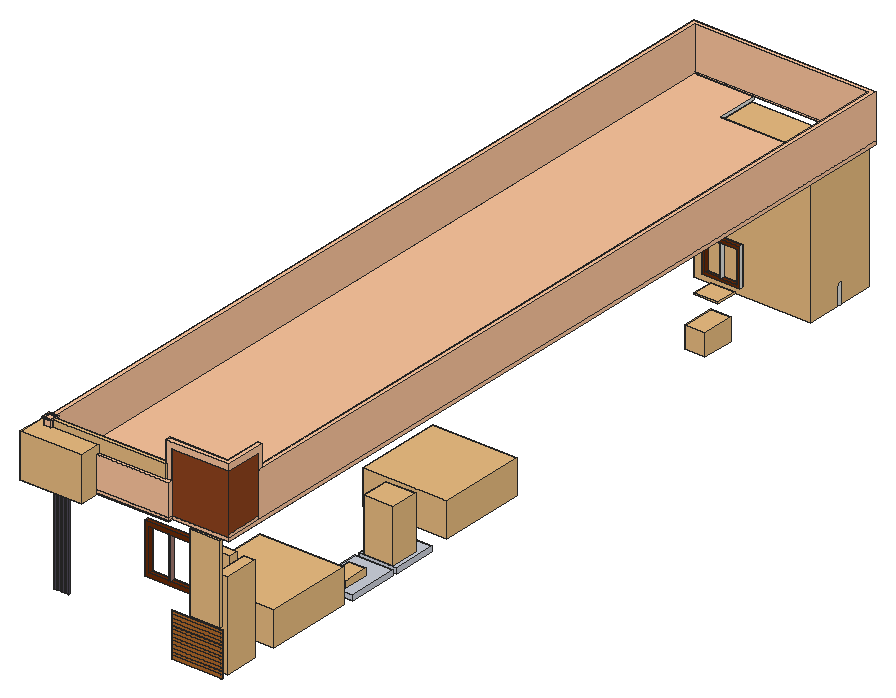
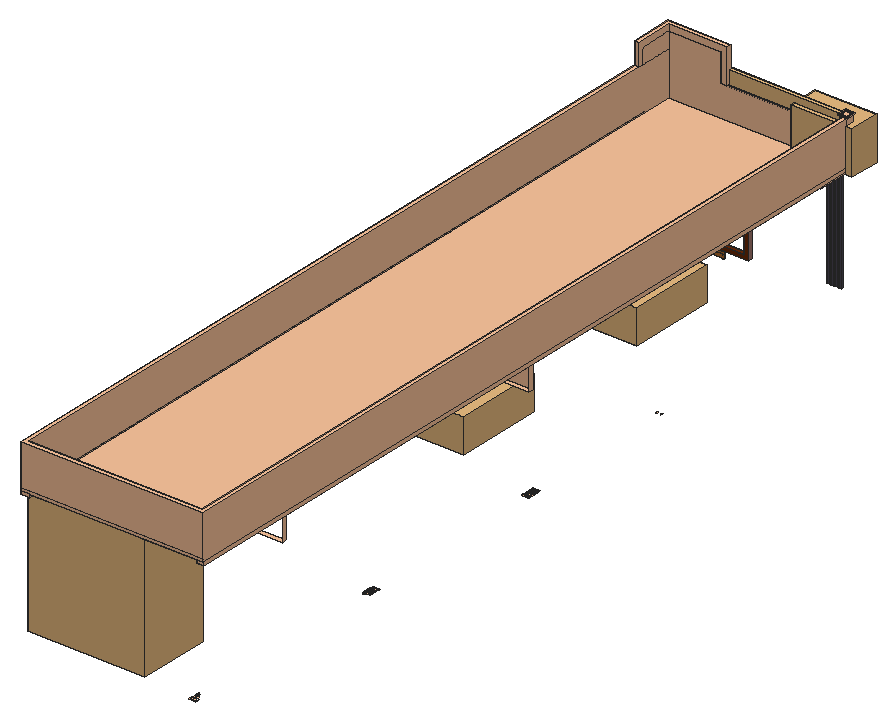
# SketchUp Ruby script. Lengths in inches.
U = 1.inch
M = Sketchup.active_model
def pt(a) = Geom::Point3d.new(a.map { |v| v * U })
def face(e, loops, mat)
  f = e.add_face(loops[0].map { |a| pt(a) })
  loops[1..].each { |l| e.add_face(l.map { |a| pt(a) }).erase! }
  f.material = f.back_material = mat if mat
  f
end
# faces: each face lists its corners as indices into pts; further lists are holes
def faces(e, pts, list, mat = nil) = list.each { |f| face(e, (f[0].is_a?(Array) ? f : [f]).map { |l| l.map { |i| pts[i] } }, mat) }
# xy, xz, yz: faces in a plane at the given z, y or x. An outline is a flat list of corners, or four numbers for a rectangle; further outlines are holes
def ring(l) = l.size == 4 ? [[l[0], l[1]], [l[2], l[1]], [l[2], l[3]], [l[0], l[3]]] : l.each_slice(2).to_a
def flat(e, list, mat, &to3) = list.each { |f| face(e, (f[0].is_a?(Array) ? f : [f]).map { |l| ring(l).map { |u, v| to3.(u, v) } }, mat) }
def xy(e, z, list, mat = nil) = flat(e, list, mat) { |x, y| [x, y, z] }
def xz(e, y, list, mat = nil) = flat(e, list, mat) { |x, z| [x, y, z] }
def yz(e, x, list, mat = nil) = flat(e, list, mat) { |y, z| [x, y, z] }
def lines(e, pts, list) = list.each { |a, b| e.add_line(pt(pts[a]), pt(pts[b])) }
# prism: a flat outline (further loops are holes) pulled along v
def prism(e, loops, v, mat = nil)
  f = face(e, loops, mat); d = Geom::Vector3d.new(v.map { |x| x * U })
  f.pushpull(f.normal.samedirection?(d) ? d.length : -d.length)
end
def box(e, o, s, mat = nil) = prism(e, [[o, [o[0] + s[0], o[1], o[2]], [o[0] + s[0], o[1] + s[1], o[2]], [o[0], o[1] + s[1], o[2]]]], [0, 0, s[2]], mat)
def at(x, y, z, deg = 0) = Geom::Transformation.translation(pt([x, y, z])) * Geom::Transformation.rotation(ORIGIN, Z_AXIS, deg.degrees)
def axes(o, x, y, z) = Geom::Transformation.new([*x, 0, *y, 0, *z, 0, *pt(o).to_a, 1])
def part(name) = M.definitions.add(name)
# library, detail: a bought-in or finely detailed component or shape, given as its bounding box
def library(name, o, s) = part(name).tap { |d| box(d.entities, o, s) }
def detail(e, o, s) = box(e.add_group.entities, o, s)
def put(e, d, t, mat = nil) = e.add_instance(d, t).tap { |i| i.material = mat if mat }
def group(e, t, mat = nil) = e.add_group.tap { |g| g.transformation = t; g.material = mat if mat }.entities
root = M.entities
M.materials.add("[0023_FireBrick]").color = [178, 34, 34]
M.materials.add("[Color A01]1").color = [163, 122, 112]
M.materials.add("[Color A02]1").color = [252, 197, 157]
M.materials.add("[Color M06]").color = [77, 72, 86]
M.materials.add("[Marble Carrara Floor Tile]").color = [204, 208, 219]
M.materials.add("[Wood Bamboo]").color = [177, 105, 43]
M.materials.add("[Wood Fence]1").color = [142, 67, 30]
M.materials.add("[Wood Veneer 02]").color = [107, 42, 7]
c1 = part("Group\#210")
box(c1.entities,[0,0,-0.3125],[36.0625,48,5.3125])
c2 = library("Group\#15",[-0.01,-1.53,0.79],[112.05,69.48,120])
c3 = library("Double bed",[0,0,0],[90.55,83.75,32.69])
c4 = part("Component\#5")
box(c4.entities,[0,-0.625,0],[48.6875,0.625,3.09])
c5 = library("P2 Single Open Right",[0,0,0],[8.91,82.42,82.52])
c6 = library("Group\#135",[0,0,0],[10.8125,33,84])
c7 = library("Squat+Toilet",[-7.87,-3.06,-5.41],[15.8,23.9,6.66])
c8 = library("My Toilet",[37.42,56.99,0],[19.17,25.6,30.6])
c9 = part("Frame upright")
box(c9.entities,[0,0,-39.22],[3.05,1.4,102],"[Color M06]")
c10 = library("Sink with faucet",[0,-0.57,-6.81],[19.24,30.87,20.8])
c11 = library("2-TABLE DE CUISSON CLC2",[-11.42,-10.04,0],[22.84,20.08,1.26])
c12 = part("Group87\#1")
xy(c12.entities,0,[[[-24,-24,24,24],[0.59,-20.0625,20.0625,20.0625],[-20.0625,-20.0625,-0.59,20.0625]]],"[Wood Veneer 02]")
xy(c12.entities,5.875,[[[-24,-24,24,24],[0.59,-20.0625,20.0625,20.0625],[-20.0625,-20.0625,-0.59,20.0625]]],"[Wood Veneer 02]")
xz(c12.entities,-24,[[-24,0,24,5.875]])
xz(c12.entities,-20.0625,[[-20.0625,0,-0.59,5.875],[0.59,0,20.0625,5.875]],"[Wood Veneer 02]")
xz(c12.entities,20.0625,[[-20.0625,0,-0.59,5.875],[0.59,0,20.0625,5.875]])
xz(c12.entities,24,[[-24,0,24,5.875]],"[Wood Veneer 02]")
yz(c12.entities,-24,[[-24,0,24,5.875]])
yz(c12.entities,-20.0625,[[-20.0625,0,20.0625,5.875]],"[Wood Veneer 02]")
yz(c12.entities,-0.59,[[-20.0625,0,20.0625,5.875]],"[Wood Veneer 02]")
yz(c12.entities,0.59,[[-20.0625,0,20.0625,5.875]])
yz(c12.entities,20.0625,[[-20.0625,0,20.0625,5.875]],"[Wood Veneer 02]")
yz(c12.entities,24,[[-24,0,24,5.875]])
c13 = library("jali",[235.9375,0,0],[159,318,2])
c14 = library("ARTIFICIAL VINES & FLOWERS",[-442.26,-138.3125,250.52],[58.45,28.9,41.46])
c15 = part("Square post")
box(c15.entities,[0,0,0],[7.1875,7.1875,27.41])
c16 = part("Component\#11")
xy(c16.entities,0,[[0,0,7.1875,7.1875]])
xy(c16.entities,12.79,[[[-0.9,-0.9,8.09,8.09],[0,0,7.1875,7.1875]],[0,0,7.1875,7.1875]])
xy(c16.entities,13.54,[[[-0.9,-0.9,8.09,8.09],[0,0,7.1875,7.1875]]])
xz(c16.entities,-0.9,[[-0.9,12.79,8.09,13.54]])
xz(c16.entities,0,[[0,0,7.1875,12.79],[0,12.79,7.1875,13.54]])
xz(c16.entities,7.1875,[[0,0,7.1875,12.79],[0,12.79,7.1875,13.54]])
xz(c16.entities,8.09,[[-0.9,12.79,8.09,13.54]])
yz(c16.entities,-0.9,[[-0.9,12.79,8.09,13.54]])
yz(c16.entities,0,[[0,0,7.1875,12.79],[0,12.79,7.1875,13.54]])
yz(c16.entities,7.1875,[[0,0,7.1875,12.79],[0,12.79,7.1875,13.54]])
yz(c16.entities,8.09,[[-0.9,12.79,8.09,13.54]])
c17 = library("Group\#181",[0,0,0],[107.67,3.9375,12.79])
box(root,[98.75,741.65,131.89],[75.61,3.31,19.68])
xy(root,131.89,[[11.25,222.37,12.14,223.25,11.26,224.13,10.36,223.26],[15.65,223.28,15.84,223.47,15.84,224.86,15.65,225.05,14.77,224.16],[15.84,224.86,15.84,225.24,15.65,225.05],[8.88,372.26,9.13,372.26,9.51,372.64,8.88,373.27],[9.13,372.26,9.89,372.26,9.51,372.64],
  [9.89,372.26,10.9,372.26,11.28,372.64,10.4,373.52,9.51,372.64],[10.9,372.26,11.66,372.26,11.28,372.64],[11.66,372.26,12.42,372.26,12.42,373.27,12.17,373.52,11.28,372.64],[12.42,372.26,12.68,372.26,13.06,372.64,12.42,373.27],[12.68,372.26,13.4375,372.26,13.06,372.64],
  [13.4375,372.26,14.45,372.26,14.83,372.64,13.94,373.52,13.06,372.64],[14.45,372.26,15.21,372.26,14.83,372.64],[15.21,372.26,15.84,372.26,15.84,373.27,15.65,373.46,14.83,372.64],[11.28,372.64,12.17,373.52,11.28,374.41,10.4,373.52],[13.06,372.64,13.94,373.52,13.06,374.41,12.42,373.78,12.42,373.27],
  [14.83,372.64,15.65,373.46,14.78,374.36,13.94,373.52],[12.42,373.27,12.42,373.78,12.17,373.52],[15.84,373.27,15.84,373.65,15.65,373.46],[15.65,373.46,15.84,373.65,15.84,375.04,15.65,375.23,14.78,374.36],[10.4,373.52,11.28,374.41,10.4,375.3,9.51,374.41],
  [12.17,373.52,12.42,373.78,12.42,375.04,12.17,375.3,11.28,374.41],[13.94,373.52,14.78,374.36,13.9,375.25,13.06,374.41],[8.88,373.78,9.51,374.41,8.88,375.04],[12.42,373.78,13.06,374.41,12.42,375.04],[14.78,374.36,15.65,375.23,14.78,376.13,13.9,375.25],
  [9.51,374.41,10.4,375.3,9.51,376.18,8.88,375.55,8.88,375.04],[11.28,374.41,12.17,375.3,11.28,376.18,10.4,375.3],[13.06,374.41,13.9,375.25,13.02,376.14,12.42,375.55,12.42,375.04],[12.42,375.04,12.42,375.55,12.17,375.3],[15.84,375.04,15.84,375.42,15.65,375.23],
  [15.65,375.23,15.84,375.42,15.84,376.82,15.65,377.01,14.78,376.13],[13.9,375.25,14.78,376.13,13.9,377.02,13.02,376.14],[10.4,375.3,11.28,376.18,10.4,377.07,9.51,376.18],[12.17,375.3,12.42,375.55,12.42,376.75,12.14,377.04,11.28,376.18],[8.88,375.55,9.51,376.18,8.88,376.82],
  [12.42,375.55,13.02,376.14,12.42,376.75],[14.78,376.13,15.65,377.01,14.78,377.9,13.9,377.02],[9.51,376.18,10.4,377.07,9.51,377.95,8.88,377.32,8.88,376.82],[11.28,376.18,12.14,377.04,11.26,377.93,10.4,377.07],[15.65,377.01,15.84,377.19,15.84,378.59,15.65,378.78,14.78,377.9],
  [13.9,377.02,14.78,377.9,13.9,378.8,13.02,377.92],[12.14,377.04,12.42,377.32,12.42,378.52,12.14,378.8125,11.26,377.93],[10.4,377.07,11.26,377.93,10.38,378.83,9.51,377.95],[8.88,377.32,9.51,377.95,8.88,378.59],[12.42,377.32,13.02,377.92,12.42,378.52],
  [14.78,377.9,15.65,378.78,14.78,379.67,13.9,378.8],[13.02,377.92,13.9,378.8,13.02,379.69,12.42,379.09,12.42,378.52],[11.26,377.93,12.14,378.8125,11.26,379.71,10.38,378.83],[9.51,377.95,10.38,378.83,9.51,379.72,8.88,379.09,8.88,378.59],[15.65,378.78,15.84,378.97,15.84,380.36,15.66,380.55,14.78,379.67],
  [13.9,378.8,14.78,379.67,13.9,380.57,13.02,379.69],[12.14,378.8125,12.42,379.09,12.42,380.3,12.14,380.58,11.26,379.71],[10.38,378.83,11.26,379.71,10.38,380.6,9.51,379.72],[8.88,379.09,9.51,379.72,8.88,380.36],[12.42,379.09,13.02,379.69,12.42,380.3],
  [14.78,379.67,15.66,380.55,14.78,381.45,13.9,380.57],[9.51,379.72,10.38,380.6,9.51,381.49,8.88,380.87,8.88,380.36],[13.9,380.57,14.78,381.45,13.91,382.35,13.02,381.46],[12.14,380.58,12.42,380.87,12.42,382.07,12.14,382.36,11.26,381.48],[14.78,381.45,15.66,382.33,14.79,383.23,13.91,382.35],
  [13.02,381.46,13.91,382.35,13.03,383.25,12.42,382.64,12.42,382.07],[12.42,382.07,12.42,382.64,12.14,382.36],[15.66,382.33,15.84,382.51,15.84,383.91,15.66,384.11,14.79,383.23],[13.91,382.35,14.79,383.23,13.92,384.14,13.03,383.25],[12.14,382.36,12.42,382.64,12.42,383.87,12.16,384.14,11.27,383.25],
  [10.38,382.37,11.27,383.25,10.39,384.15,9.51,383.27],[12.42,382.64,13.03,383.25,12.42,383.87],[14.79,383.23,15.66,384.11,14.82,385.03,13.92,384.14],[11.27,383.25,12.16,384.14,11.28,385.04,10.39,384.15],[13.03,383.25,13.92,384.14,13.05,385.04,12.42,384.41,12.42,383.87],
  [9.51,383.27,10.39,384.15,9.51,385.04,8.88,384.41,8.88,383.91],[12.42,383.87,12.42,384.41,12.16,384.14],[15.66,384.11,15.84,384.29,15.84,385.3,15.08,385.3,14.82,385.03],[12.16,384.14,12.42,384.41,12.42,385.3,11.54,385.3,11.28,385.04],[13.92,384.14,14.82,385.03,14.58,385.3,13.31,385.3,13.05,385.04],
  [10.39,384.15,11.28,385.04,11.03,385.3,9.76,385.3,9.51,385.04],[8.88,384.41,9.51,385.04,9.26,385.3,8.88,385.3],[12.42,384.41,13.05,385.04,12.8,385.3,12.42,385.3],[8.88,564.35,9.13,564.35,9.51,564.73,8.88,565.36],[9.13,564.35,9.89,564.35,9.51,564.73],
  [9.89,564.35,10.9,564.35,11.28,564.73,10.4,565.62,9.51,564.73],[10.9,564.35,11.66,564.35,11.28,564.73],[11.66,564.35,12.42,564.35,12.42,565.36,12.17,565.62,11.28,564.73],[12.42,564.35,12.68,564.35,13.06,564.73,12.42,565.36],[12.68,564.35,13.4375,564.35,13.06,564.73],
  [13.4375,564.35,14.45,564.35,14.83,564.73,13.94,565.62,13.06,564.73],[14.45,564.35,15.21,564.35,14.83,564.73],[9.51,564.73,10.4,565.62,9.51,566.5,8.88,565.87,8.88,565.36],[11.28,564.73,12.17,565.62,11.28,566.5,10.4,565.62],[13.06,564.73,13.94,565.62,13.06,566.5,12.42,565.87,12.42,565.36],
  [13.94,565.62,14.78,566.45,13.9,567.34,13.06,566.5],[8.88,565.87,9.51,566.5,8.88,567.14],[12.42,565.87,13.06,566.5,12.42,567.14],[14.78,566.45,15.65,567.33,14.77,568.21,13.9,567.34],[9.51,566.5,10.4,567.39,9.51,568.28,8.88,567.64,8.88,567.14],
  [13.06,566.5,13.9,567.34,13.02,568.24,12.42,567.64,12.42,567.14],[15.65,567.33,15.84,567.52,15.84,568.91,15.65,569.1,14.77,568.21],[13.9,567.34,14.77,568.21,13.88,569.1,13.02,568.24],[10.4,567.39,11.28,568.28,10.4,569.16,9.51,568.28],[12.17,567.39,12.42,567.64,12.42,568.85,12.14,569.13,11.28,568.28],
  [8.88,567.64,9.51,568.28,8.88,568.91],[12.42,567.64,13.02,568.24,12.42,568.85],[14.77,568.21,15.65,569.1,14.77,569.99,13.88,569.1],[13.02,568.24,13.88,569.1,12.99,569.99,12.42,569.42,12.42,568.85],[9.51,568.28,10.4,569.16,9.51,570.05,8.88,569.42,8.88,568.91],
  [11.28,568.28,12.14,569.13,11.26,570.03,10.4,569.16],[12.42,568.85,12.42,569.42,12.14,569.13],[13.88,569.1,14.77,569.99,13.88,570.87,12.99,569.99],[15.65,569.1,15.84,569.29,15.84,570.68,15.65,570.87,14.77,569.99],[12.14,569.13,12.42,569.42,12.42,570.56,12.11,570.87,11.26,570.03],
  [10.4,569.16,11.26,570.03,10.38,570.92,9.51,570.05],[8.88,569.42,9.51,570.05,8.88,570.68],[12.42,569.42,12.99,569.99,12.42,570.56],[12.99,569.99,13.88,570.87,12.99,571.76,12.42,571.1875,12.42,570.56],[14.77,569.99,15.65,570.87,14.77,571.76,13.88,570.87],
  [11.26,570.03,12.11,570.87,11.22,571.76,10.38,570.92],[9.51,570.05,10.38,570.92,9.51,571.81,8.88,571.1875,8.88,570.68],[12.11,570.87,12.42,571.1875,12.42,572.33,12.11,572.65,11.22,571.76],[13.88,570.87,14.77,571.76,13.88,572.65,12.99,571.76],[10.38,570.92,11.22,571.76,10.35,572.63,9.51,571.81],
  [8.88,571.1875,9.51,571.81,8.88,572.46],[12.42,571.1875,12.99,571.76,12.42,572.33],[11.22,571.76,12.11,572.65,11.25,573.51,10.35,572.63],[12.99,571.76,13.88,572.65,12.99,573.53,12.42,572.96,12.42,572.33],[14.77,571.76,15.65,572.65,14.77,573.53,13.88,572.65],
  [9.51,571.81,10.35,572.63,9.46,573.52,8.88,572.96,8.88,572.46],[12.42,572.33,12.42,572.96,12.11,572.65],[10.35,572.63,11.25,573.51,10.36,574.4,9.46,573.52],[12.11,572.65,12.42,572.96,12.42,574.1,12.14,574.38,11.25,573.51],[13.88,572.65,14.77,573.53,13.88,574.42,12.99,573.53],
  [15.65,572.65,15.84,572.84,15.84,574.23,15.65,574.42,14.77,573.53],[8.88,572.96,9.46,573.52,8.88,574.1],[12.42,572.96,12.99,573.53,12.42,574.1],[11.25,573.51,12.14,574.38,11.26,575.27,10.36,574.4],[9.46,573.52,10.36,574.4,9.46,575.29,8.88,574.73,8.88,574.1],
  [12.99,573.53,13.88,574.42,13.04,575.26,12.42,574.66,12.42,574.1],[14.77,573.53,15.65,574.42,14.77,575.3,13.88,574.42],[12.42,574.1,12.42,574.66,12.14,574.38],[12.14,574.38,12.42,574.66,12.42,575.875,12.15,576.14,11.26,575.27],[13.88,574.42,14.77,575.3,13.93,576.14,13.04,575.26],
  [15.65,574.42,15.84,574.61,15.84,576,15.65,576.19,14.77,575.3],[12.42,574.66,13.04,575.26,12.42,575.875],[13.04,575.26,13.93,576.14,13.05,577.02,12.42,576.41,12.42,575.875],[14.77,575.3,15.65,576.19,14.83,577.02,13.93,576.14],[13.93,576.14,14.83,577.02,14.58,577.27,13.31,577.27,13.05,577.02],
  [15.84,771.51,15.84,771.89,15.66,771.7],[15.66,771.7,15.84,771.89,15.84,773.29,15.66,773.47,14.79,772.57],[15.84,773.29,15.84,773.67,15.66,773.47],[13.91,773.45,14.78,774.35,13.94,775.1875,13.06,774.3],[15.66,773.47,15.84,773.67,15.84,775.06,15.66,775.25,15.84,775.44,15.84,776.83,15.72,776.96,14.83,776.07,15.66,775.25,14.78,774.35],
  [15.84,775.06,15.84,775.44,15.66,775.25],[15.84,776.83,15.84,777.09,15.72,776.96],[12.17,776.96,13.06,777.85,12.17,778.73,11.28,777.85],[13.94,776.96,14.83,777.85,15.72,778.73,14.83,779.62,15.66,780.45,14.79,781.35,13.94,780.51,13.06,781.39,13.92,782.25,13.05,783.16,13.92,782.25,14.79,781.35,13.94,780.51,15.84,778.61,15.84,777.09,15.72,776.96,14.83,777.85,13.94,778.73,13.06,777.85],[15.72,776.96,15.84,777.09,15.84,778.61,15.72,778.73,14.83,777.85],
  [15.84,778.61,15.84,778.86,15.72,778.73],[13.06,779.62,13.94,780.51,12.17,782.28,11.28,783.16,9.51,781.39,8.88,782.02,8.88,780.76,10.4,782.28,11.28,781.39,13.05,783.16,13.92,782.25,14.82,783.15,14.58,783.42,13.31,783.42,12.17,782.28,13.06,781.39,12.17,780.51],[15.84,780.25,15.84,780.63,15.66,780.45],[15.66,782.22,15.84,782.4,15.84,783.42,15.08,783.42,14.82,783.15],[9.51,783.16,9.76,783.42,9.26,783.42],
  [11.28,783.16,11.54,783.42,11.03,783.42],[13.05,783.16,13.31,783.42,12.8,783.42]],"[Color A02]1")
xy(root,167.89,[[104.48,665.91,140.48,670.34]],"[Color A02]1")
xy(root,203.89,[[104.48,665.91,140.48,670.34]],"[Color A02]1")
xy(root,215.89,[[126.53,46.0625,150.53,50.62],[52.9375,119.63,57.37,155.6],[82.95,164.21,87.38,194.22],[57.37,258.67,77.375,263.23],[16.86,371.24,52.9375,375.68],
  [57.37,371.24,83.33,375.68],[96.37,573.85,126.38,578.28],[16.86,665.91,64.84,670.34]],"[Color A02]1")
xy(root,251.89,[[0.9,46.0625,7.87,784.43],[52.9375,46.0625,156.53,46.0625,156.53,50.62,57.37,50.62,57.37,119.63,52.9375,119.63],[156.53,46.0625,166.9,50.62],[171.33,61,175.89,61,175.89,212.21,171.33,212.21,171.33,164.21,52.9375,164.21,52.9375,119.63,57.37,119.63,57.37,160.15,171.33,160.15],[82.95,164.21,87.38,164.21,87.38,212.2,166.89,212.2,166.89,216.63,57.37,216.63,57.37,375.68,16.86,375.68,16.86,371.24,52.9375,371.24,52.9375,212.2,82.95,212.2],
  [171.33,227.14,175.89,227.14,175.89,371.25,171.33,371.25,171.33,263.23,57.37,263.23,57.37,258.67,171.33,258.67],[57.37,371.24,166.9,375.68],[7.87,386.1875,12.42,563.34],[171.33,386.1875,175.89,563.34],[87.89,573.85,166.9,573.85,166.9,578.28,92.44,578.28,92.44,665.91,171.33,665.91,171.33,578.28,175.89,578.28,175.89,670.34,16.86,670.34,16.86,665.91,87.89,665.91],
  [7.87,578.28,12.42,578.28,12.42,665.91,16.86,665.91,16.86,670.34,7.87,670.34]],"[Color A02]1")
xz(root,371.24,[[16.86,215.89,52.9375,251.89]],"[Color A02]1")
yz(root,16.86,[[371.24,215.89,375.68,251.89],[665.91,215.89,670.34,251.89]],"[Color A02]1")
yz(root,104.48,[[665.91,167.89,670.34,203.89]],"[Color A02]1")
yz(root,140.48,[[665.91,167.89,670.34,203.89]],"[Color A02]1")
p = [[169.9,779.32,257.89],[6.9,779.32,257.89],[169.9,46.0625,257.89],[175.89,785.32,257.89],[0.9,785.32,257.89],[107.4375,669.12,170.88],
  [122.04,669.12,170.88],[110.75,50.62,171.82],[110.75,50.62,211.95],[91.28,50.62,171.82],[91.28,50.62,211.95],[70.625,50.62,211.95],
  [70.625,50.62,171.82],[90.09,50.62,211.95],[90.09,50.62,171.82]]
lines(root,p,[[0,1],[2,0],[3,4],[5,6],[7,8],[9,7],[10,9],[8,10],[11,12],[13,11],[14,13],[12,14]])
put(root,c1,at(135.46,164.2,132.2),"[Marble Carrara Floor Tile]")
put(root,c1,axes([135.46,216.63,132.2],[1,0,0],[0,0.87583,0],[0,0,1]),"[Marble Carrara Floor Tile]")
put(root,c2,at(62.29,710.41,131.1))
put(root,c3,axes([167.8125,281.22,132.26],[-0.89,0,0],[0,1,0],[0,0,1]))
put(root,c3,axes([171.125,70.44,132.26],[-0.89,0,0],[0,1,0],[0,0,1]))
put(root,c4,at(121.89,10.0625,132.5),"[Wood Bamboo]")
put(root,c5,axes([150.59,43.27,133.39],[0,1,0],[-0.3,0,0],[0,0,1]))
put(root,c6,at(161.9,13.0625,135.04))
put(root,c4,at(121.89,10.0625,135.68),"[Wood Bamboo]")
put(root,c7,at(153.05,171.69,142.3))
put(root,c8,axes([223.82,302.41,137.85],[-1.48104,0,0],[0,-1.04,0],[0,0,1.65]))
put(root,c4,at(121.89,10.0625,138.87),"[Wood Bamboo]")
put(root,c4,at(121.89,10.0625,142.06),"[Wood Bamboo]")
put(root,c4,at(121.89,10.0625,145.25),"[Wood Bamboo]")
put(root,c4,at(121.89,10.0625,148.43),"[Wood Bamboo]")
g1 = group(root,at(5.65,14.01,149.89))
put(g1,c9,at(0,0,39.22))
put(g1,c9,at(3.75,0,39.22))
put(g1,c9,at(11.4375,0,39.22))
put(g1,c9,at(7.5,0,39.22))
put(root,c4,at(121.89,10.0625,151.62),"[Wood Bamboo]")
put(root,c4,at(121.89,10.0625,154.81),"[Wood Bamboo]")
put(root,c10,at(152.21,586.64,162.18))
put(root,c4,at(121.89,10.0625,158),"[Wood Bamboo]")
put(root,c4,at(121.89,10.0625,161.18),"[Wood Bamboo]")
put(root,c11,at(123.65,656.6875,161.89))
put(root,c4,at(121.89,10.0625,164.37),"[Wood Bamboo]")
put(root,c4,at(121.89,10.0625,167.56),"[Wood Bamboo]")
put(root,c12,axes([90.6875,50.62,191.89],[1,0,0],[0,0,1],[0,-0.72,0]),"[Color A01]1")
put(root,c12,axes([122.48,669.12,186.125],[0.75,0,0],[0,0,0.76],[0,-0.5472,0]))
put(root,c4,at(121.89,10.0625,170.73),"[Wood Bamboo]")
put(root,c13,axes([98.13,9.125,176.82],[0.18169,0,0],[0,0,0.23605],[0,-1.01,0]))
put(root,c14,at(436.24,126.71,0))
g2 = group(root,at(0.88,6.0625,0))
g3 = group(g2,at(0,0,0))
xy(g3,251.07,[[0.01,0,0.01,40,15.96,40,15.96,728.43,26.63,728.43,26.63,10.67,110.33,10.67,110.33,29.33,41.375,29.33,41.375,728.43,52.04,728.43,52.04,40,121,40,121,0]],"[Color A02]1")
xy(g3,251.89,[[0.01,0,121,0,121,40,52.04,40,52.04,728.43,41.375,728.43,41.375,29.33,110.33,29.33,110.33,10.67,26.63,10.67,26.63,728.43,15.96,728.43,15.96,40,0.01,40],[121,4,121,40,52.04,40,52.04,728.43,61.39,728.43,61.39,734.68,131.41,734.68,131.41,774.75,166.24,774.75,166.24,779.25,175.01,779.25,175.01,4],[0,24.89,0.01,40],[0.01,40,0.01,778.37,6.96,778.37,6.96,774.75,61.39,774.75,61.39,728.43,15.96,728.43,15.96,40]],"[Color A02]1")
xy(g3,253.01,[[26.63,10.67,26.63,728.43,41.375,728.43,41.375,29.33,110.33,29.33,110.33,10.67]],"[0023_FireBrick]")
xy(g3,255.07,[[0.01,0,121,0,121,4,175.01,4,175.01,779.25,166.24,779.25,166.24,774.75,131.41,774.75,131.41,734.68,61.39,734.68,61.39,774.75,6.96,774.75,6.96,778.37,0.01,778.37]],"[Color A02]1")
xz(g3,0,[[0.01,251.07,121,251.89],[0.01,251.89,121,255.07]],"[Color A02]1")
xz(g3,4,[[121,251.89,175.01,255.07]],"[Color A02]1")
xz(g3,10.67,[[26.63,251.07,110.33,251.89],[26.63,251.89,110.33,253.01]],"[Color A02]1")
xz(g3,29.33,[[41.375,251.07,110.33,251.89],[41.375,251.89,110.33,253.01]],"[Color A02]1")
xz(g3,40,[[0.01,251.07,15.96,251.89],[52.04,251.07,121,251.89]],"[Color A02]1")
xz(g3,728.43,[[26.63,251.89,41.375,253.01],[41.375,251.89,61.39,253.01]])
xz(g3,728.43,[[15.96,251.07,26.63,251.89],[26.63,251.07,41.375,251.89],[41.375,251.07,52.04,251.89]],"[Color A02]1")
xz(g3,734.68,[[61.39,251.89,131.41,255.07]])
xz(g3,774.75,[[131.41,251.89,166.24,255.07]])
xz(g3,774.75,[[6.96,251.89,61.39,255.07]],"[Color A02]1")
xz(g3,778.37,[[0.01,251.89,6.96,255.07]],"[Color A02]1")
xz(g3,779.25,[[166.24,251.89,175.01,255.07]],"[Color A02]1")
yz(g3,0.01,[[0,251.07,24.89,251.89],[24.89,251.07,40,251.89],[0,251.89,778.37,255.07]],"[Color A02]1")
yz(g3,6.96,[[774.75,251.89,778.37,255.07]],"[Color A02]1")
yz(g3,15.96,[[40,251.07,728.43,251.89]],"[Color A02]1")
yz(g3,26.63,[[10.67,251.07,728.43,251.89],[10.67,251.89,728.43,253.01]],"[Color A02]1")
yz(g3,41.375,[[29.33,251.07,728.43,251.89],[29.33,251.89,728.43,253.01]],"[Color A02]1")
yz(g3,52.04,[[40,251.07,728.43,251.89]],"[Color A02]1")
yz(g3,61.39,[[728.43,251.89,734.68,253.01],[734.68,251.89,774.75,255.07]])
yz(g3,110.33,[[10.67,251.07,29.33,251.89],[10.67,251.89,29.33,253.01]],"[Color A02]1")
yz(g3,121,[[0,251.07,4,251.89],[4,251.07,40,251.89],[0,251.89,4,255.07]],"[Color A02]1")
yz(g3,131.41,[[734.68,251.89,774.75,255.07]])
yz(g3,166.24,[[774.75,251.89,779.25,255.07]],"[Color A02]1")
yz(g3,175.01,[[4,251.89,779.25,255.07]],"[Color A02]1")
put(root,c15,at(0.9,6.0625,255.07),"[Color A02]1")
g4 = group(root,at(0.9,6.0625,255.07))
xy(g4,0,[[[39.17,0,39.17,4,0,4,0,779.25,174.99,779.25,174.99,4,120.99,4,120.99,0],[4.5,8.5,170.5,774.75]]],"[Color A02]1")
xy(g4,27.41,[[0,0,39.17,4]],"[Color A02]1")
xy(g4,30.125,[[0,0,120.99,0,120.99,4,114.99,4,114.99,8.5,0,8.5],[114.99,4,120.99,8.5]],"[Color A02]1")
xy(g4,42.125,[[0,8.5,4.5,8.5,4.5,774.75,170.5,774.75,170.5,44.375,174.99,44.375,174.99,779.25,0,779.25]],"[Color A02]1")
xy(g4,57.05,[[120.99,4,174.99,4,174.99,40,170.5,40,170.5,8.5,120.99,8.5]],"[Color A02]1")
xy(g4,63.05,[[114.99,4,174.99,4,174.99,44.375,170.5,44.375,170.5,8.5,114.99,8.5]],"[Color A02]1")
xz(g4,0,[[39.17,0,120.99,30.125],[0,27.41,39.17,30.125]],"[Color A02]1")
xz(g4,4,[[0,0,39.17,27.41],[114.99,30.125,120.99,30.125,120.99,57.05,174.99,57.05,174.99,63.05,114.99,63.05]],"[Color A02]1")
xz(g4,4,[[120.99,0,174.99,57.05]],"[Wood Fence]1")
xz(g4,8.5,[[4.5,0,4.5,30.125,120.99,30.125,120.99,57.05,170.5,57.05,170.5,0],[0,30.125,4.5,42.125],[114.99,30.125,114.99,63.05,170.5,63.05,170.5,57.05,120.99,57.05,120.99,30.125]],"[Color A02]1")
xz(g4,40,[[170.5,42.125,174.99,57.05]],"[Color A02]1")
xz(g4,44.375,[[170.5,42.125,174.99,63.05]],"[Color A02]1")
xz(g4,774.75,[[4.5,0,170.5,42.125]],"[Color A02]1")
xz(g4,779.25,[[0,0,174.99,42.125]],"[Color A02]1")
yz(g4,0,[[4,0,4,27.41,0,27.41,0,30.125,8.5,30.125,8.5,42.125,779.25,42.125,779.25,0]],"[Color A02]1")
yz(g4,4.5,[[8.5,0,774.75,42.125]],"[Color A02]1")
yz(g4,39.17,[[0,0,4,27.41]],"[Color A02]1")
yz(g4,114.99,[[4,30.125,8.5,63.05]],"[Color A02]1")
yz(g4,120.99,[[0,0,4,30.125],[4,30.125,8.5,57.05]],"[Color A02]1")
yz(g4,170.5,[[8.5,0,774.75,42.125],[40,42.125,40,57.05,8.5,57.05,8.5,63.05,44.375,63.05,44.375,42.125],[8.5,42.125,40,57.05]],"[Color A02]1")
yz(g4,174.99,[[4,0,40,2.8125],[40,0,779.25,42.125],[40,42.125,44.375,42.125,44.375,63.05,4,63.05,4,57.05,40,57.05]],"[Color A02]1")
yz(g4,174.99,[[4,2.8125,40,57.05]],"[Wood Fence]1")
put(root,c16,at(0.9,7.375,285.2),"[Color A02]1")
put(root,c17,axes([8.3,9,285.2],[1.01,0,0],[0,1,0],[0,0,1]))
